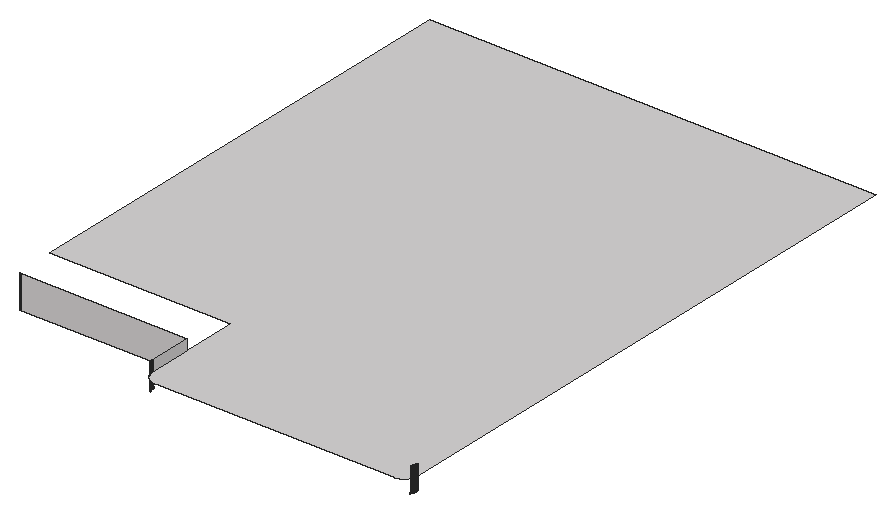
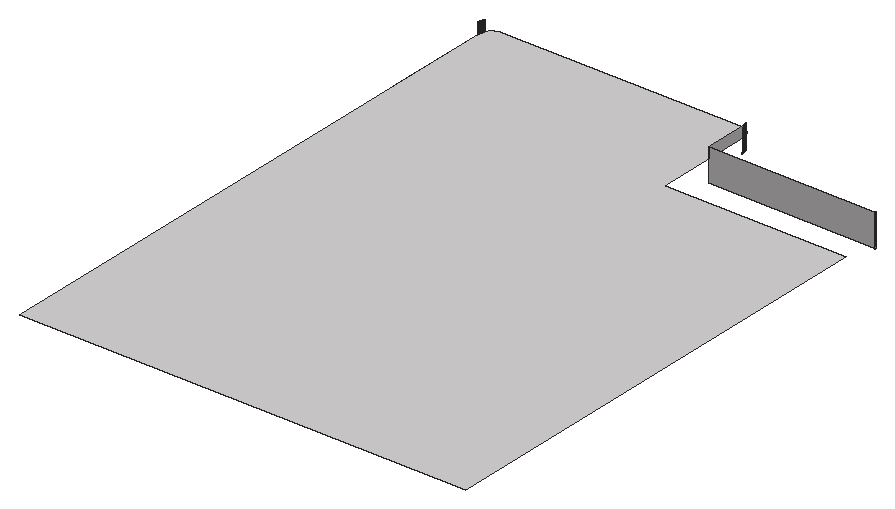
# SketchUp Ruby script. Lengths in inches.
U = 1.inch
M = Sketchup.active_model
def pt(a) = Geom::Point3d.new(a.map { |v| v * U })
def face(e, loops, mat)
  f = e.add_face(loops[0].map { |a| pt(a) })
  loops[1..].each { |l| e.add_face(l.map { |a| pt(a) }).erase! }
  f.material = f.back_material = mat if mat
  f
end
# faces: each face lists its corners as indices into pts; further lists are holes
def faces(e, pts, list, mat = nil) = list.each { |f| face(e, (f[0].is_a?(Array) ? f : [f]).map { |l| l.map { |i| pts[i] } }, mat) }
# xy, xz, yz: faces in a plane at the given z, y or x. An outline is a flat list of corners, or four numbers for a rectangle; further outlines are holes
def ring(l) = l.size == 4 ? [[l[0], l[1]], [l[2], l[1]], [l[2], l[3]], [l[0], l[3]]] : l.each_slice(2).to_a
def flat(e, list, mat, &to3) = list.each { |f| face(e, (f[0].is_a?(Array) ? f : [f]).map { |l| ring(l).map { |u, v| to3.(u, v) } }, mat) }
def xy(e, z, list, mat = nil) = flat(e, list, mat) { |x, y| [x, y, z] }
def xz(e, y, list, mat = nil) = flat(e, list, mat) { |x, z| [x, y, z] }
def yz(e, x, list, mat = nil) = flat(e, list, mat) { |y, z| [x, y, z] }
def lines(e, pts, list) = list.each { |a, b| e.add_line(pt(pts[a]), pt(pts[b])) }
# prism: a flat outline (further loops are holes) pulled along v
def prism(e, loops, v, mat = nil)
  f = face(e, loops, mat); d = Geom::Vector3d.new(v.map { |x| x * U })
  f.pushpull(f.normal.samedirection?(d) ? d.length : -d.length)
end
def box(e, o, s, mat = nil) = prism(e, [[o, [o[0] + s[0], o[1], o[2]], [o[0] + s[0], o[1] + s[1], o[2]], [o[0], o[1] + s[1], o[2]]]], [0, 0, s[2]], mat)
def at(x, y, z, deg = 0) = Geom::Transformation.translation(pt([x, y, z])) * Geom::Transformation.rotation(ORIGIN, Z_AXIS, deg.degrees)
def axes(o, x, y, z) = Geom::Transformation.new([*x, 0, *y, 0, *z, 0, *pt(o).to_a, 1])
def part(name) = M.definitions.add(name)
# library, detail: a bought-in or finely detailed component or shape, given as its bounding box
def library(name, o, s) = part(name).tap { |d| box(d.entities, o, s) }
def detail(e, o, s) = box(e.add_group.entities, o, s)
def put(e, d, t, mat = nil) = e.add_instance(d, t).tap { |i| i.material = mat if mat }
def group(e, t, mat = nil) = e.add_group.tap { |g| g.transformation = t; g.material = mat if mat }.entities
root = M.entities
M.materials.add("[Quartz Light Brown]").color = [215, 212, 212]
xy(root,384,[[216,143,215.804,143.001,215.607,143.005,215.411,143.012,215.215,143.021,215.019,143.032,214.823,143.046,214.627,143.063,214.432,143.082,214.237,143.104,214.042,143.128,213.848,143.155,213.653,143.185,213.46,143.217,213.266,143.251,213.074,143.288,212.881,143.328,212.69,143.37,212.498,143.414,212.308,143.462,212.118,143.511,211.928,143.563,211.74,143.618,211.552,143.675,211.365,143.734,211.178,143.796,210.993,143.86,210.808,143.927,210.624,143.996,210.442,144.068,210.26,144.142,210.079,144.218,209.899,144.297,209.72,144.378,209.542,144.461,209.366,144.547,209.19,144.635,209.016,144.725,208.843,144.818,208.671,144.913,208.5,145.01,208.331,145.109,208.163,145.21,207.996,145.314,207.83,145.42,207.666,145.528,207.504,145.638,207.343,145.75,207.183,145.865,207.025,145.981,206.869,146.1,206.714,146.22,206.56,146.343,206.408,146.467,206.258,146.594,206.11,146.722,205.963,146.853,205.818,146.985,205.675,147.119,205.533,147.255,205.393,147.393,205.255,147.533,205.119,147.675,204.985,147.818,204.853,147.963,204.722,148.11,204.594,148.258,204.467,148.408,204.343,148.56,204.22,148.714,204.1,148.869,203.981,149.025,203.865,149.183,203.75,149.343,203.638,149.504,203.528,149.666,203.42,149.83,203.314,149.996,203.21,150.163,203.109,150.331,203.01,150.5,202.913,150.671,202.818,150.843,202.725,151.016,202.635,151.19,202.547,151.366,202.461,151.542,202.378,151.72,202.297,151.899,202.218,152.079,202.142,152.26,202.068,152.442,201.996,152.624,201.927,152.808,201.86,152.993,201.796,153.178,201.734,153.365,201.675,153.552,201.618,153.74,201.563,153.928,201.511,154.118,201.462,154.308,201.414,154.498,201.37,154.69,201.328,154.881,201.288,155.074,201.251,155.266,201.217,155.46,201.185,155.653,201.155,155.848,201.128,156.042,201.104,156.237,201.082,156.432,201.063,156.627,201.046,156.823,201.032,157.019,201.021,157.215,201.012,157.411,201.005,157.607,201.001,157.804,201,158,201,266,0,266,0,794,495,794,495,158,494.999,157.804,494.995,157.607,494.988,157.411,494.979,157.215,494.968,157.019,494.954,156.823,494.937,156.627,494.918,156.432,494.896,156.237,494.872,156.042,494.845,155.848,494.815,155.653,494.783,155.46,494.749,155.266,494.712,155.074,494.672,154.881,494.63,154.69,494.586,154.498,494.538,154.308,494.489,154.118,494.437,153.928,494.382,153.74,494.325,153.552,494.266,153.365,494.204,153.178,494.14,152.993,494.073,152.808,494.004,152.624,493.932,152.442,493.858,152.26,493.782,152.079,493.703,151.899,493.622,151.72,493.539,151.542,493.453,151.366,493.365,151.19,493.275,151.016,493.182,150.843,493.087,150.671,492.99,150.5,492.891,150.331,492.79,150.163,492.686,149.996,492.58,149.83,492.472,149.666,492.362,149.504,492.25,149.343,492.135,149.183,492.019,149.025,491.9,148.869,491.78,148.714,491.657,148.56,491.533,148.408,491.406,148.258,491.278,148.11,491.147,147.963,491.015,147.818,490.881,147.675,490.745,147.533,490.607,147.393,490.467,147.255,490.325,147.119,490.182,146.985,490.037,146.853,489.89,146.722,489.742,146.594,489.592,146.467,489.44,146.343,489.286,146.22,489.131,146.1,488.975,145.981,488.817,145.865,488.657,145.75,488.496,145.638,488.334,145.528,488.17,145.42,488.004,145.314,487.837,145.21,487.669,145.109,487.5,145.01,487.329,144.913,487.157,144.818,486.984,144.725,486.81,144.635,486.634,144.547,486.458,144.461,486.28,144.378,486.101,144.297,485.921,144.218,485.74,144.142,485.558,144.068,485.376,143.996,485.192,143.927,485.007,143.86,484.822,143.796,484.635,143.734,484.448,143.675,484.26,143.618,484.072,143.563,483.882,143.511,483.692,143.462,483.502,143.414,483.31,143.37,483.119,143.328,482.926,143.288,482.734,143.251,482.54,143.217,482.347,143.185,482.152,143.155,481.958,143.128,481.763,143.104,481.568,143.082,481.373,143.063,481.177,143.046,480.981,143.032,480.785,143.021,480.589,143.012,480.393,143.005,480.196,143.001,480,143],[[216,143,480,143,480.196,143.001,480.393,143.005,480.589,143.012,480.785,143.021,480.981,143.032,481.177,143.046,481.373,143.063,481.568,143.082,481.763,143.104,481.958,143.128,482.152,143.155,482.347,143.185,482.54,143.217,482.734,143.251,482.926,143.288,483.119,143.328,483.31,143.37,483.502,143.414,483.692,143.462,483.882,143.511,484.072,143.563,484.26,143.618,484.448,143.675,484.635,143.734,484.822,143.796,485.007,143.86,485.192,143.927,485.376,143.996,485.558,144.068,485.74,144.142,485.921,144.218,486.101,144.297,486.28,144.378,486.458,144.461,486.634,144.547,486.81,144.635,486.984,144.725,487.157,144.818,487.329,144.913,487.5,145.01,487.669,145.109,487.837,145.21,488.004,145.314,488.17,145.42,488.334,145.528,488.496,145.638,488.657,145.75,488.817,145.865,488.975,145.981,489.131,146.1,489.286,146.22,489.44,146.343,489.592,146.467,489.742,146.594,489.89,146.722,490.037,146.853,490.182,146.985,490.325,147.119,490.467,147.255,490.607,147.393,490.745,147.533,490.881,147.675,491.015,147.818,491.147,147.963,491.278,148.11,491.406,148.258,491.533,148.408,491.657,148.56,491.78,148.714,491.9,148.869,492.019,149.025,492.135,149.183,492.25,149.343,492.362,149.504,492.472,149.666,492.58,149.83,492.686,149.996,492.79,150.163,492.891,150.331,492.99,150.5,493.087,150.671,493.182,150.843,493.275,151.016,493.365,151.19,493.453,151.366,493.539,151.542,493.622,151.72,493.703,151.899,493.782,152.079,493.858,152.26,493.932,152.442,494.004,152.624,494.073,152.808,494.14,152.993,494.204,153.178,494.266,153.365,494.325,153.552,494.382,153.74,494.437,153.928,494.489,154.118,494.538,154.308,494.586,154.498,494.63,154.69,494.672,154.881,494.712,155.074,494.749,155.266,494.783,155.46,494.815,155.653,494.845,155.848,494.872,156.042,494.896,156.237,494.918,156.432,494.937,156.627,494.954,156.823,494.968,157.019,494.979,157.215,494.988,157.411,494.995,157.607,494.999,157.804,495,158,495,275,492,275,492,794,0,794,0,266,201,266,201,158,201.001,157.804,201.005,157.607,201.012,157.411,201.021,157.215,201.032,157.019,201.046,156.823,201.063,156.627,201.082,156.432,201.104,156.237,201.128,156.042,201.155,155.848,201.185,155.653,201.217,155.46,201.251,155.266,201.288,155.074,201.328,154.881,201.37,154.69,201.414,154.498,201.462,154.308,201.511,154.118,201.563,153.928,201.618,153.74,201.675,153.552,201.734,153.365,201.796,153.178,201.86,152.993,201.927,152.808,201.996,152.624,202.068,152.442,202.142,152.26,202.218,152.079,202.297,151.899,202.378,151.72,202.461,151.542,202.547,151.366,202.635,151.19,202.725,151.016,202.818,150.843,202.913,150.671,203.01,150.5,203.109,150.331,203.21,150.163,203.314,149.996,203.42,149.83,203.528,149.666,203.638,149.504,203.75,149.343,203.865,149.183,203.981,149.025,204.1,148.869,204.22,148.714,204.343,148.56,204.467,148.408,204.594,148.258,204.722,148.11,204.853,147.963,204.985,147.818,205.119,147.675,205.255,147.533,205.393,147.393,205.533,147.255,205.675,147.119,205.818,146.985,205.963,146.853,206.11,146.722,206.258,146.594,206.408,146.467,206.56,146.343,206.714,146.22,206.869,146.1,207.025,145.981,207.183,145.865,207.343,145.75,207.504,145.638,207.666,145.528,207.83,145.42,207.996,145.314,208.163,145.21,208.331,145.109,208.5,145.01,208.671,144.913,208.843,144.818,209.016,144.725,209.19,144.635,209.366,144.547,209.542,144.461,209.72,144.378,209.899,144.297,210.079,144.218,210.26,144.142,210.442,144.068,210.624,143.996,210.808,143.927,210.993,143.86,211.178,143.796,211.365,143.734,211.552,143.675,211.74,143.618,211.928,143.563,212.118,143.511,212.308,143.462,212.498,143.414,212.69,143.37,212.881,143.328,213.074,143.288,213.266,143.251,213.46,143.217,213.653,143.185,213.848,143.155,214.042,143.128,214.237,143.104,214.432,143.082,214.627,143.063,214.823,143.046,215.019,143.032,215.215,143.021,215.411,143.012,215.607,143.005,215.804,143.001],[215.961,155,215.921,155.001,215.882,155.002,215.879,155.002,215.843,155.004,215.804,155.006,215.765,155.009,215.761,155.01,215.725,155.013,215.686,155.016,215.647,155.021,215.644,155.021,215.608,155.026,215.57,155.031,215.531,155.037,215.528,155.037,215.492,155.043,215.453,155.05,215.415,155.058,215.412,155.058,215.376,155.066,215.338,155.074,215.3,155.083,215.297,155.084,215.262,155.092,215.224,155.102,215.186,155.113,215.183,155.113,215.148,155.124,215.11,155.135,215.073,155.147,215.07,155.148,215.036,155.159,214.962,155.185,214.959,155.186,214.925,155.199,214.888,155.214,214.852,155.228,214.85,155.229,214.816,155.244,214.78,155.259,214.744,155.276,214.742,155.277,214.708,155.292,214.673,155.309,214.638,155.327,214.636,155.328,214.603,155.345,214.569,155.364,214.534,155.383,214.532,155.384,214.5,155.402,214.466,155.422,214.433,155.442,214.431,155.443,214.399,155.463,214.366,155.484,214.333,155.506,214.332,155.507,214.301,155.528,214.269,155.55,214.237,155.573,214.235,155.574,214.205,155.596,214.143,155.644,214.142,155.645,214.082,155.693,214.052,155.719,214.051,155.72,214.022,155.744,213.993,155.771,213.964,155.797,213.963,155.798,213.935,155.824,213.907,155.851,213.851,155.907,213.824,155.935,213.797,155.964,213.796,155.965,213.771,155.993,213.744,156.022,213.719,156.052,213.693,156.082,213.669,156.112,213.644,156.143,213.596,156.205,213.55,156.269,213.506,156.333,213.484,156.366,213.463,156.399,213.442,156.433,213.422,156.466,213.402,156.5,213.383,156.534,213.364,156.569,213.345,156.603,213.309,156.673,213.292,156.708,213.276,156.744,213.259,156.78,213.244,156.816,213.228,156.852,213.214,156.888,213.199,156.925,213.185,156.962,213.159,157.036,213.135,157.11,213.102,157.224,213.092,157.262,213.074,157.338,213.066,157.376,213.058,157.415,213.05,157.453,213.043,157.492,213.031,157.57,213.026,157.608,213.016,157.686,213.013,157.725,213.009,157.765,213.006,157.804,213.004,157.843,213.003,157.881,213.002,157.882,213.001,157.921,213,157.961,213,275,9,275,9,785,483,785,483,157.961,482.999,157.921,482.998,157.882,482.996,157.846,482.996,157.843,482.994,157.804,482.991,157.765,482.988,157.735,482.988,157.729,482.987,157.725,482.984,157.686,482.979,157.647,482.976,157.623,482.976,157.617,482.975,157.613,482.974,157.608,482.969,157.57,482.963,157.531,482.96,157.512,482.959,157.504,482.958,157.497,482.957,157.492,482.95,157.453,482.942,157.415,482.94,157.401,482.9375,157.391,482.936,157.382,482.934,157.376,482.926,157.338,482.917,157.3,482.915,157.29,482.909,157.268,482.908,157.262,482.898,157.224,482.887,157.186,482.886,157.18,482.883,157.168,482.878,157.155,482.876,157.148,482.865,157.11,482.853,157.073,482.853,157.071,482.849,157.058,482.843,157.043,482.841,157.036,482.828,156.999,482.816,156.967,482.815,156.962,482.811,156.95,482.804,156.932,482.801,156.925,482.786,156.888,482.777,156.864,482.772,156.852,482.768,156.843,482.76,156.823,482.756,156.816,482.741,156.78,482.732,156.762,482.724,156.744,482.722,156.738,482.711,156.716,482.708,156.708,482.691,156.673,482.684,156.661,482.673,156.638,482.672,156.635,482.659,156.61,482.655,156.603,482.636,156.569,482.632,156.561,482.602,156.507,482.598,156.5,482.578,156.466,482.576,156.462,482.56,156.435,482.558,156.433,482.541,156.405,482.537,156.399,482.516,156.366,482.498,156.338,482.494,156.333,482.476,156.306,482.472,156.301,482.46,156.283,482.45,156.269,482.433,156.244,482.427,156.237,482.406,156.209,482.404,156.205,482.397,156.196,482.38,156.174,482.364,156.152,482.356,156.143,482.333,156.114,482.331,156.112,482.329,156.109,482.307,156.082,482.291,156.063,482.281,156.052,482.256,156.022,482.229,155.993,482.216,155.976,482.203,155.964,482.176,155.935,482.149,155.907,482.137,155.893,482.121,155.879,482.093,155.851,482.065,155.824,482.054,155.813,482.036,155.797,482.007,155.771,481.978,155.744,481.969,155.736,481.948,155.719,481.918,155.693,481.888,155.669,481.881,155.662,481.857,155.644,481.795,155.596,481.791,155.592,481.763,155.573,481.731,155.55,481.699,155.528,481.697,155.525,481.667,155.506,481.634,155.484,481.601,155.463,481.567,155.442,481.534,155.422,481.503,155.403,481.5,155.402,481.466,155.383,481.431,155.364,481.403,155.347,481.397,155.345,481.327,155.309,481.3,155.295,481.292,155.292,481.256,155.276,481.22,155.259,481.196,155.248,481.184,155.244,481.148,155.228,481.112,155.214,481.09,155.204,481.075,155.199,481.038,155.185,481.001,155.172,480.982,155.164,480.964,155.159,480.89,155.135,480.873,155.129,480.852,155.124,480.776,155.102,480.762,155.098,480.738,155.092,480.662,155.074,480.651,155.071,480.624,155.066,480.585,155.058,480.547,155.05,480.538,155.048,480.508,155.043,480.43,155.031,480.425,155.029,480.392,155.026,480.314,155.016,480.311,155.015,480.275,155.013,480.235,155.009,480.196,155.006,480.118,155.002,480.082,155,480.079,155.001,216,155]]],"[Quartz Light Brown]")
xz(root,205,[[18,360,201,396]],"[Quartz Light Brown]")
yz(root,201,[[158,384,205,396]],"[Quartz Light Brown]")
p = [[16.823,205.039,396],[16.588,205.055,396],[16.588,205.055,360],[16.823,205.039,360],[17.058,205.025,396],[17.058,205.025,360],
  [17.293,205.014,396],[17.293,205.014,360],[17.529,205.006,396],[17.529,205.006,360],[17.764,205.002,396],[17.764,205.002,360],
  [18,205,396],[18,205,360],[15.884,205.125,396],[15.651,205.154,396],[15.651,205.154,360],[15.884,205.125,360],
  [16.118,205.099,396],[16.118,205.099,360],[16.353,205.076,396],[16.353,205.076,360],[15.417,205.186,396],[15.417,205.186,360],
  [203.785,151.159,369],[203.785,151.159,368],[203.876,151,368],[203.876,151,369],[492.124,151,369],[492.124,151,368],
  [492.215,151.159,368],[492.215,151.159,369],[203.697,151.32,369],[203.697,151.32,368],[492.303,151.32,368],[492.303,151.32,369],
  [203.61,151.481,369],[203.61,151.481,368],[492.39,151.481,368],[492.39,151.481,369],[203.526,151.644,369],[203.526,151.644,368],
  [492.474,151.644,368],[492.474,151.644,369],[203.444,151.808,369],[203.444,151.808,368],[492.556,151.808,368],[492.556,151.808,369],
  [203.364,151.973,369],[203.364,151.973,368],[492.636,151.973,368],[492.636,151.973,369],[203.286,152.139,369],[203.286,152.139,368],
  [492.714,152.139,368],[492.714,152.139,369],[203.21,152.306,369],[203.21,152.306,368],[492.79,152.306,368],[492.79,152.306,369],
  [203.137,152.474,369],[203.137,152.474,368],[492.863,152.474,368],[492.863,152.474,369],[203.066,152.642,369],[203.066,152.642,368],
  [492.934,152.642,368],[492.934,152.642,369],[202.997,152.812,369],[202.997,152.812,368],[493.003,152.812,368],[493.003,152.812,369],
  [202.93,152.983,369],[202.93,152.983,368],[493.07,152.983,368],[493.07,152.983,369],[202.865,153.154,369],[202.865,153.154,368],
  [493.135,153.154,368],[493.135,153.154,369],[202.803,153.327,369],[202.803,153.327,368],[493.197,153.327,368],[493.197,153.327,369],
  [202.743,153.5,369],[202.743,153.5,368],[493.257,153.5,368],[493.257,153.5,369],[202.685,153.674,369],[202.685,153.674,368],
  [493.315,153.674,368],[493.315,153.674,369],[202.63,153.848,369],[202.63,153.848,368],[493.37,153.848,368],[493.37,153.848,369],
  [202.577,154.024,369],[202.577,154.024,368],[493.423,154.024,368],[493.423,154.024,369],[202.526,154.2,369],[202.526,154.2,368],
  [493.474,154.2,368],[493.474,154.2,369],[202.477,154.377,369],[202.477,154.377,368],[493.523,154.377,368],[493.523,154.377,369],
  [202.431,154.554,369],[202.431,154.554,368],[493.569,154.554,368],[493.569,154.554,369],[202.387,154.732,369],[202.387,154.732,368],
  [493.613,154.732,368],[493.613,154.732,369],[202.345,154.91,369],[202.345,154.91,368],[493.655,154.91,368],[493.655,154.91,369],
  [202.306,155.089,369],[202.306,155.089,368],[493.694,155.089,368],[493.694,155.089,369],[202.269,155.269,369],[202.269,155.269,368],
  [493.731,155.269,368],[493.731,155.269,369],[202.234,155.449,369],[202.234,155.449,368],[493.766,155.449,368],[493.766,155.449,369],
  [202.202,155.629,369],[202.202,155.629,368],[493.798,155.629,368],[493.798,155.629,369],[202.172,155.81,369],[202.172,155.81,368],
  [493.828,155.81,368],[493.828,155.81,369],[202.145,155.991,369],[202.145,155.991,368],[493.855,155.991,368],[493.855,155.991,369],
  [202.12,156.173,369],[202.12,156.173,368],[493.88,156.173,368],[493.88,156.173,369],[202.097,156.354,369],[202.097,156.354,368],
  [493.903,156.354,368],[493.903,156.354,369],[202.077,156.537,369],[202.077,156.537,368],[493.923,156.537,368],[493.923,156.537,369],
  [202.059,156.719,369],[202.059,156.719,368],[493.941,156.719,368],[493.941,156.719,369],[202.043,156.902,369],[202.043,156.902,368],
  [493.957,156.902,368],[493.957,156.902,369],[202.03,157.084,369],[202.03,157.084,368],[493.97,157.084,368],[493.97,157.084,369],
  [202.019,157.267,369],[202.019,157.267,368],[493.981,157.267,368],[493.981,157.267,369],[202.011,157.45,369],[202.011,157.45,368],
  [493.989,157.45,368],[493.989,157.45,369],[202.005,157.634,369],[202.005,157.634,368],[493.995,157.634,368],[493.995,157.634,369],
  [202.001,157.817,369],[202.001,157.817,368],[493.999,157.817,368],[493.999,157.817,369],[202,158.003,369],[202,158.003,368],
  [494,158.003,368],[494,158.003,369],[202.818,150.843,384],[202.725,151.016,384],[202.725,151.016,369],[202.818,150.843,369],
  [493.275,151.016,384],[493.182,150.843,384],[493.182,150.843,369],[493.275,151.016,369],[202.635,151.19,384],[202.635,151.19,369],
  [493.365,151.19,384],[493.365,151.19,369],[202.547,151.366,384],[202.547,151.366,369],[493.453,151.366,384],[493.453,151.366,369],
  [202.461,151.542,384],[202.461,151.542,369],[493.539,151.542,384],[493.539,151.542,369],[202.378,151.72,384],[202.378,151.72,369],
  [493.622,151.72,384],[493.622,151.72,369],[202.297,151.899,384],[202.297,151.899,369],[493.703,151.899,384],[493.703,151.899,369],
  [202.218,152.079,384],[202.218,152.079,369],[493.782,152.079,384],[493.782,152.079,369],[202.142,152.26,384],[202.142,152.26,369],
  [493.858,152.26,384],[493.858,152.26,369],[202.068,152.442,384],[202.068,152.442,369],[493.932,152.442,384],[493.932,152.442,369],
  [201.996,152.624,384],[201.996,152.624,369],[494.004,152.624,384],[494.004,152.624,369],[201.927,152.808,384],[201.927,152.808,369],
  [494.073,152.808,384],[494.073,152.808,369],[201.86,152.993,384],[201.86,152.993,369],[494.14,152.993,384],[494.14,152.993,369],
  [201.796,153.178,384],[201.796,153.178,369],[494.204,153.178,384],[494.204,153.178,369],[201.734,153.365,384],[201.734,153.365,369],
  [494.266,153.365,384],[494.266,153.365,369],[201.675,153.552,384],[201.675,153.552,369],[494.325,153.552,384],[494.325,153.552,369],
  [201.618,153.74,384],[201.618,153.74,369],[494.382,153.74,384],[494.382,153.74,369],[201.563,153.928,384],[201.563,153.928,369],
  [494.437,153.928,384],[494.437,153.928,369],[201.511,154.118,384],[201.511,154.118,369],[494.489,154.118,384],[494.489,154.118,369],
  [201.462,154.308,384],[201.462,154.308,369],[494.538,154.308,384],[494.538,154.308,369],[201.414,154.498,384],[201.414,154.498,369],
  [494.586,154.498,384],[494.586,154.498,369],[201.37,154.69,384],[201.37,154.69,369],[494.63,154.69,384],[494.63,154.69,369],
  [201.328,154.881,384],[201.328,154.881,369],[494.672,154.881,384],[494.672,154.881,369],[201.288,155.074,384],[201.288,155.074,369],
  [494.712,155.074,384],[494.712,155.074,369],[201.251,155.266,384],[201.251,155.266,369],[494.749,155.266,384],[494.749,155.266,369],
  [201.217,155.46,384],[201.217,155.46,369],[494.783,155.46,384],[494.783,155.46,369],[201.185,155.653,384],[201.185,155.653,369],
  [494.815,155.653,384],[494.815,155.653,369],[201.155,155.848,384],[201.155,155.848,369],[494.845,155.848,384],[494.845,155.848,369],
  [201.128,156.042,384],[201.128,156.042,369],[494.872,156.042,384],[494.872,156.042,369],[201.104,156.237,384],[201.104,156.237,369],
  [494.896,156.237,384],[494.896,156.237,369],[201.082,156.432,384],[201.082,156.432,369],[494.918,156.432,384],[494.918,156.432,369],
  [201.063,156.627,384],[201.063,156.627,369],[494.937,156.627,384],[494.937,156.627,369],[201.046,156.823,384],[201.046,156.823,369],
  [494.954,156.823,384],[494.954,156.823,369],[201.032,157.019,384],[201.032,157.019,369],[494.968,157.019,384],[494.968,157.019,369],
  [201.021,157.215,384],[201.021,157.215,369],[494.979,157.215,384],[494.979,157.215,369],[201.012,157.411,384],[201.012,157.411,369],
  [494.988,157.411,384],[494.988,157.411,369],[201.005,157.607,384],[201.005,157.607,369],[494.995,157.607,384],[494.995,157.607,369],
  [201.001,157.804,384],[201.001,157.804,369],[494.999,157.804,384],[494.999,157.804,369],[201,158,384],[201,158,369],
  [495,158,384],[495,158,369],[202.818,150.843,396],[202.725,151.016,396],[202.725,151.016,384],[202.818,150.843,384],
  [493.182,150.843,384],[493.275,151.016,384],[493.275,151.016,396],[493.182,150.843,396],[202.635,151.19,396],[202.635,151.19,384],
  [493.365,151.19,384],[493.365,151.19,396],[202.547,151.366,396],[202.547,151.366,384],[493.453,151.366,384],[493.453,151.366,396],
  [202.461,151.542,396],[202.461,151.542,384],[493.539,151.542,384],[493.539,151.542,396],[202.378,151.72,396],[202.378,151.72,384],
  [493.622,151.72,384],[493.622,151.72,396],[202.297,151.899,396],[202.297,151.899,384],[493.703,151.899,384],[493.703,151.899,396],
  [202.218,152.079,396],[202.218,152.079,384],[493.782,152.079,384],[493.782,152.079,396],[202.142,152.26,396],[202.142,152.26,384],
  [493.858,152.26,384],[493.858,152.26,396],[202.068,152.442,396],[202.068,152.442,384],[493.932,152.442,384],[493.932,152.442,396],
  [201.996,152.624,396],[201.996,152.624,384],[494.004,152.624,384],[494.004,152.624,396],[201.927,152.808,396],[201.927,152.808,384],
  [494.073,152.808,384],[494.073,152.808,396],[201.86,152.993,396],[201.86,152.993,384],[494.14,152.993,384],[494.14,152.993,396],
  [201.796,153.178,396],[201.796,153.178,384],[494.204,153.178,384],[494.204,153.178,396],[201.734,153.365,396],[201.734,153.365,384],
  [494.266,153.365,384],[494.266,153.365,396],[201.675,153.552,396],[201.675,153.552,384],[494.325,153.552,384],[494.325,153.552,396],
  [201.618,153.74,396],[201.618,153.74,384],[494.382,153.74,384],[494.382,153.74,396],[201.563,153.928,396],[201.563,153.928,384],
  [494.437,153.928,384],[494.437,153.928,396],[201.511,154.118,396],[201.511,154.118,384],[494.489,154.118,384],[494.489,154.118,396],
  [201.462,154.308,396],[201.462,154.308,384],[494.538,154.308,384],[494.538,154.308,396],[201.414,154.498,396],[201.414,154.498,384],
  [494.586,154.498,384],[494.586,154.498,396],[201.37,154.69,396],[201.37,154.69,384],[494.63,154.69,384],[494.63,154.69,396],
  [201.328,154.881,396],[201.328,154.881,384],[494.672,154.881,384],[494.672,154.881,396],[201.288,155.074,396],[201.288,155.074,384],
  [494.712,155.074,384],[494.712,155.074,396],[201.251,155.266,396],[201.251,155.266,384],[494.749,155.266,384],[494.749,155.266,396],
  [201.217,155.46,396],[201.217,155.46,384],[494.783,155.46,384],[494.783,155.46,396],[201.185,155.653,396],[201.185,155.653,384],
  [494.815,155.653,384],[494.815,155.653,396],[201.155,155.848,396],[201.155,155.848,384],[494.845,155.848,384],[494.845,155.848,396],
  [201.128,156.042,396],[201.128,156.042,384],[494.872,156.042,384],[494.872,156.042,396],[201.104,156.237,396],[201.104,156.237,384],
  [494.896,156.237,384],[494.896,156.237,396],[201.082,156.432,396],[201.082,156.432,384],[494.918,156.432,384],[494.918,156.432,396],
  [201.063,156.627,396],[201.063,156.627,384],[494.937,156.627,384],[494.937,156.627,396],[201.046,156.823,396],[201.046,156.823,384],
  [494.954,156.823,384],[494.954,156.823,396],[201.032,157.019,396],[201.032,157.019,384],[494.968,157.019,384],[494.968,157.019,396],
  [201.021,157.215,396],[201.021,157.215,384],[494.979,157.215,384],[494.979,157.215,396],[201.012,157.411,396],[201.012,157.411,384],
  [494.988,157.411,384],[494.988,157.411,396],[201.005,157.607,396],[201.005,157.607,384],[494.995,157.607,384],[494.995,157.607,396],
  [201.001,157.804,396],[201.001,157.804,384],[494.999,157.804,384],[494.999,157.804,396],[201,158,396],[201,158,384],
  [495,158,384],[495,158,396]]
faces(root,p,[[0,1,2,3],[4,0,3,5],[6,4,5,7],[8,6,7,9],[10,8,9,11],[12,10,11,13],[14,15,16,17],[18,14,17,19],
  [20,18,19,21],[1,20,21,2],[15,22,23,16],[24,25,26,27],[28,29,30,31],[32,33,25,24],[31,30,34,35],[36,37,33,32],
  [35,34,38,39],[40,41,37,36],[39,38,42,43],[44,45,41,40],[43,42,46,47],[48,49,45,44],[47,46,50,51],[52,53,49,48],
  [51,50,54,55],[56,57,53,52],[55,54,58,59],[60,61,57,56],[59,58,62,63],[64,65,61,60],[63,62,66,67],[68,69,65,64],
  [67,66,70,71],[72,73,69,68],[71,70,74,75],[76,77,73,72],[75,74,78,79],[80,81,77,76],[79,78,82,83],[84,85,81,80],
  [83,82,86,87],[88,89,85,84],[87,86,90,91],[92,93,89,88],[91,90,94,95],[96,97,93,92],[95,94,98,99],[100,101,97,96],
  [99,98,102,103],[104,105,101,100],[103,102,106,107],[108,109,105,104],[107,106,110,111],[112,113,109,108],[111,110,114,115],[116,117,113,112],
  [115,114,118,119],[120,121,117,116],[119,118,122,123],[124,125,121,120],[123,122,126,127],[128,129,125,124],[127,126,130,131],[132,133,129,128],
  [131,130,134,135],[136,137,133,132],[135,134,138,139],[140,141,137,136],[139,138,142,143],[144,145,141,140],[143,142,146,147],[148,149,145,144],
  [147,146,150,151],[152,153,149,148],[151,150,154,155],[156,157,153,152],[155,154,158,159],[160,161,157,156],[159,158,162,163],[164,165,161,160],
  [163,162,166,167],[168,169,165,164],[167,166,170,171],[172,173,169,168],[171,170,174,175],[176,177,173,172],[175,174,178,179],[180,181,177,176],
  [179,178,182,183],[184,185,181,180],[183,182,186,187],[188,189,190,191],[192,193,194,195],[189,196,197,190],[198,192,195,199],[196,200,201,197],
  [202,198,199,203],[200,204,205,201],[206,202,203,207],[204,208,209,205],[210,206,207,211],[208,212,213,209],[214,210,211,215],[212,216,217,213],
  [218,214,215,219],[216,220,221,217],[222,218,219,223],[220,224,225,221],[226,222,223,227],[224,228,229,225],[230,226,227,231],[228,232,233,229],
  [234,230,231,235],[232,236,237,233],[238,234,235,239],[236,240,241,237],[242,238,239,243],[240,244,245,241],[246,242,243,247],[244,248,249,245],
  [250,246,247,251],[248,252,253,249],[254,250,251,255],[252,256,257,253],[258,254,255,259],[256,260,261,257],[262,258,259,263],[260,264,265,261],
  [266,262,263,267],[264,268,269,265],[270,266,267,271],[268,272,273,269],[274,270,271,275],[272,276,277,273],[278,274,275,279],[276,280,281,277],
  [282,278,279,283],[280,284,285,281],[286,282,283,287],[284,288,289,285],[290,286,287,291],[288,292,293,289],[294,290,291,295],[292,296,297,293],
  [298,294,295,299],[296,300,301,297],[302,298,299,303],[300,304,305,301],[306,302,303,307],[304,308,309,305],[310,306,307,311],[308,312,313,309],
  [314,310,311,315],[312,316,317,313],[318,314,315,319],[316,320,321,317],[322,318,319,323],[320,324,325,321],[326,322,323,327],[324,328,329,325],
  [330,326,327,331],[328,332,333,329],[334,330,331,335],[332,336,337,333],[338,334,335,339],[336,340,341,337],[342,338,339,343],[344,345,346,347],
  [348,349,350,351],[345,352,353,346],[349,354,355,350],[352,356,357,353],[354,358,359,355],[356,360,361,357],[358,362,363,359],[360,364,365,361],
  [362,366,367,363],[364,368,369,365],[366,370,371,367],[368,372,373,369],[370,374,375,371],[372,376,377,373],[374,378,379,375],[376,380,381,377],
  [378,382,383,379],[380,384,385,381],[382,386,387,383],[384,388,389,385],[386,390,391,387],[388,392,393,389],[390,394,395,391],[392,396,397,393],
  [394,398,399,395],[396,400,401,397],[398,402,403,399],[400,404,405,401],[402,406,407,403],[404,408,409,405],[406,410,411,407],[408,412,413,409],
  [410,414,415,411],[412,416,417,413],[414,418,419,415],[416,420,421,417],[418,422,423,419],[420,424,425,421],[422,426,427,423],[424,428,429,425],
  [426,430,431,427],[428,432,433,429],[430,434,435,431],[432,436,437,433],[434,438,439,435],[436,440,441,437],[438,442,443,439],[440,444,445,441],
  [442,446,447,443],[444,448,449,445],[446,450,451,447],[448,452,453,449],[450,454,455,451],[452,456,457,453],[454,458,459,455],[456,460,461,457],
  [458,462,463,459],[460,464,465,461],[462,466,467,463],[464,468,469,465],[466,470,471,467],[468,472,473,469],[470,474,475,471],[472,476,477,473],
  [474,478,479,475],[476,480,481,477],[478,482,483,479],[480,484,485,481],[482,486,487,483],[484,488,489,485],[486,490,491,487],[488,492,493,489],
  [490,494,495,491],[492,496,497,493],[494,498,499,495]],"[Quartz Light Brown]")
